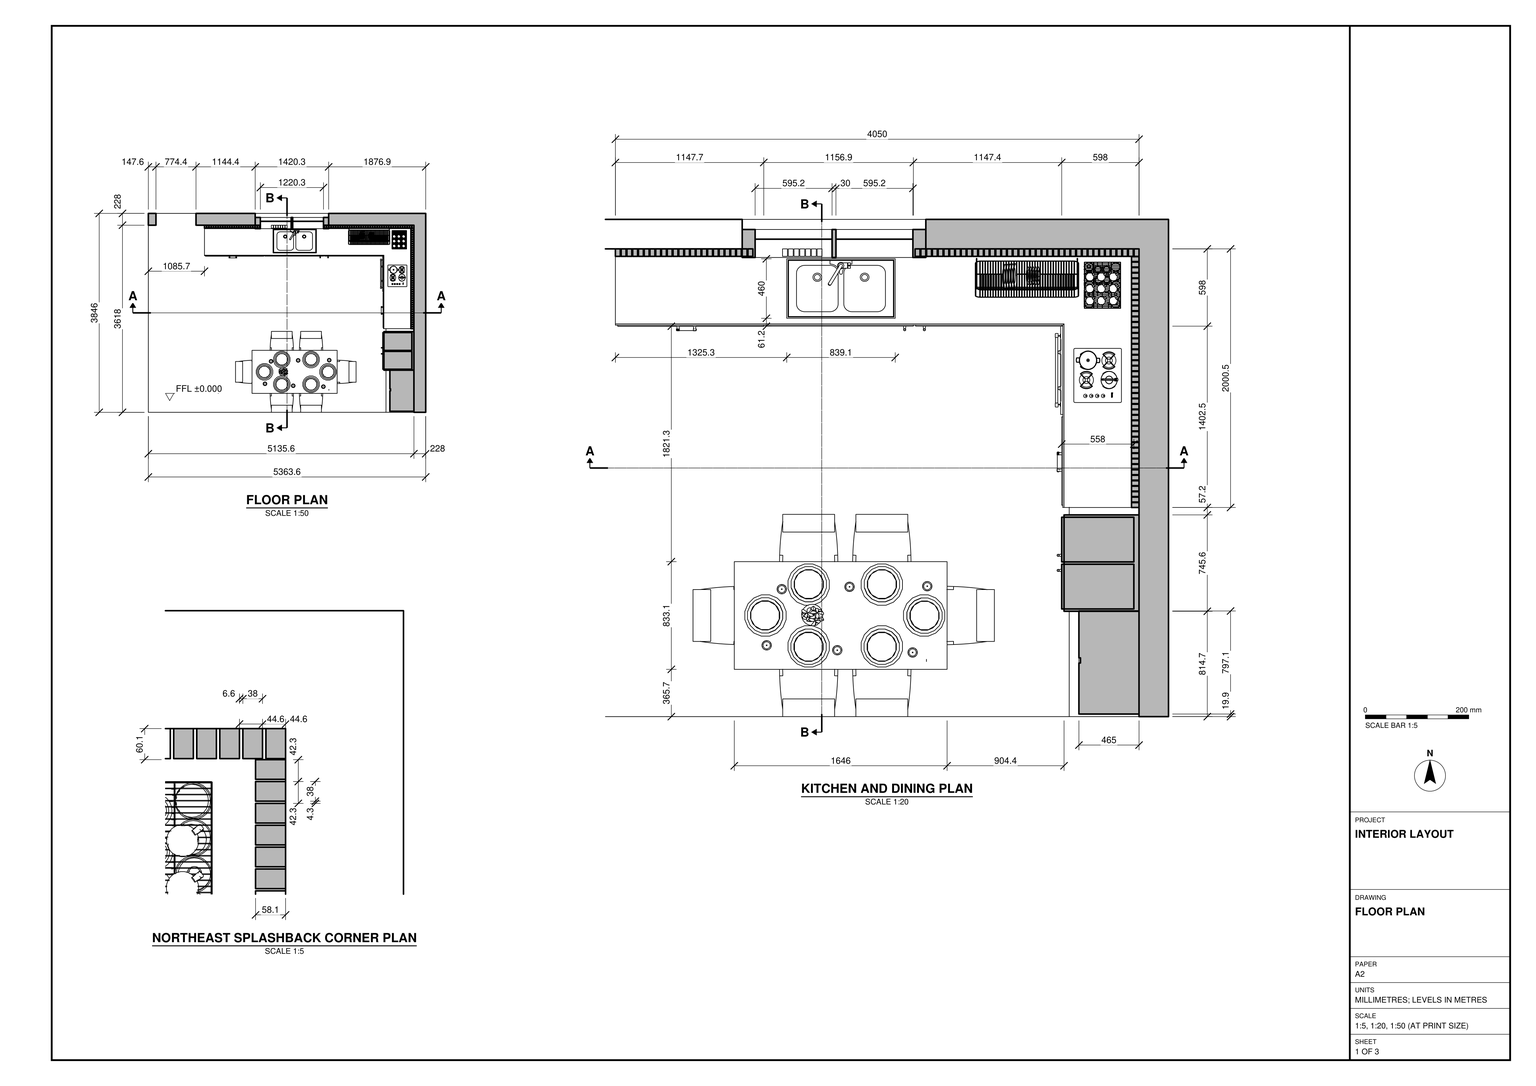
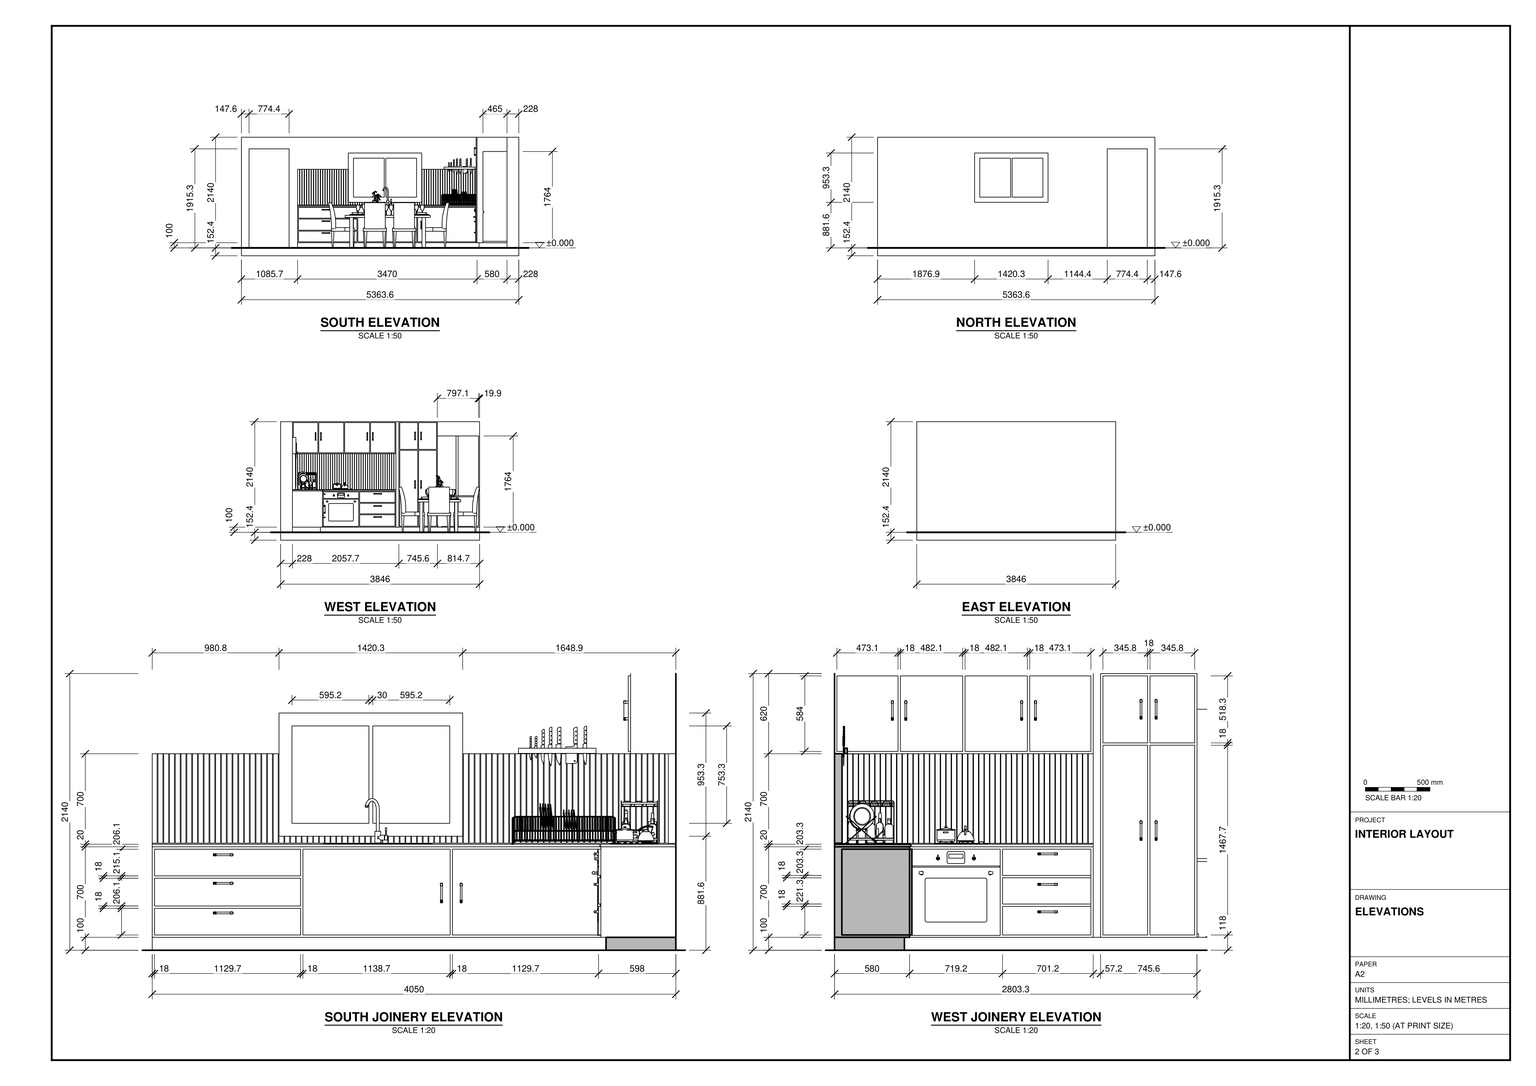
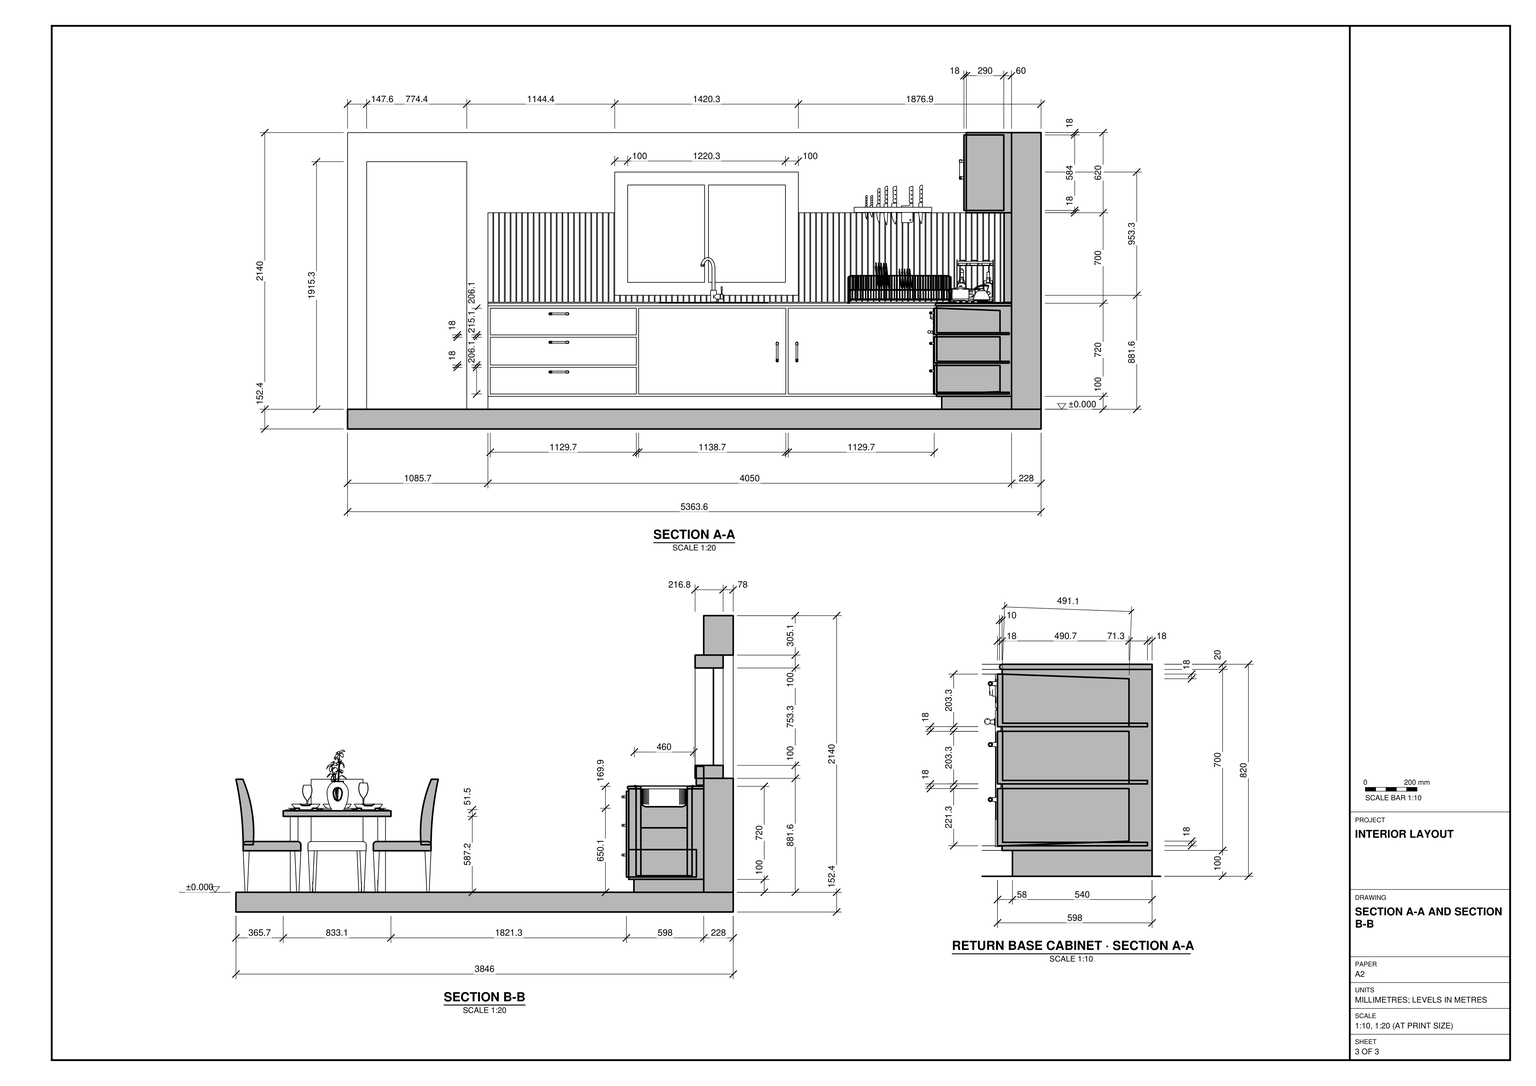
Build the kitchen and dining interior in SketchUp from task_files/diagram_01.pdf. Work in millimetres. The overall model measures 5363.6 mm east–west, 3846 mm north–south and 2292.4 mm high. Set the finished floor at 0 mm (±0.000), with the 152.4 mm slab below it. Build the 228 mm thick north and east walls to 2140 mm above the floor. Leave the south and west sides open as drawn.

Place the doorway near the west end of the north wall and the two-pane window above the double-bowl sink. Run the kitchen worktop along the north wall and turn it onto the east wall. Use the elevations and sections to lay out the plinths, drawer banks, cupboard fronts and handles. Model the vertically divided splashback around the corner, the wall cupboards above the east counter, the cooktop with the oven beneath it, and the tall storage and shallower end unit beyond the counter.

Place the rectangular dining table in the open area south of the sink, with chairs and place settings arranged as in plan. Decor, loose items and appliances may be any suitable library components. Keep the slab, walls and individual furniture and joinery pieces in separate groups or components, and use components for repeated parts. Save one SketchUp model as output_files/l_shaped_kitchen_and_six_seat_dining_area.skp.

# SketchUp Ruby script. Lengths in millimetres.
U = 1.mm
M = Sketchup.active_model
def pt(a) = Geom::Point3d.new(a.map { |v| v * U })
def face(e, loops, mat)
  f = e.add_face(loops[0].map { |a| pt(a) })
  loops[1..].each { |l| e.add_face(l.map { |a| pt(a) }).erase! }
  f.material = f.back_material = mat if mat
  f
end
# faces: each face lists its corners as indices into pts; further lists are holes
def faces(e, pts, list, mat = nil) = list.each { |f| face(e, (f[0].is_a?(Array) ? f : [f]).map { |l| l.map { |i| pts[i] } }, mat) }
# xy, xz, yz: faces in a plane at the given z, y or x. An outline is a flat list of corners, or four numbers for a rectangle; further outlines are holes
def ring(l) = l.size == 4 ? [[l[0], l[1]], [l[2], l[1]], [l[2], l[3]], [l[0], l[3]]] : l.each_slice(2).to_a
def flat(e, list, mat, &to3) = list.each { |f| face(e, (f[0].is_a?(Array) ? f : [f]).map { |l| ring(l).map { |u, v| to3.(u, v) } }, mat) }
def xy(e, z, list, mat = nil) = flat(e, list, mat) { |x, y| [x, y, z] }
def xz(e, y, list, mat = nil) = flat(e, list, mat) { |x, z| [x, y, z] }
def yz(e, x, list, mat = nil) = flat(e, list, mat) { |y, z| [x, y, z] }
def lines(e, pts, list) = list.each { |a, b| e.add_line(pt(pts[a]), pt(pts[b])) }
# prism: a flat outline (further loops are holes) pulled along v
def prism(e, loops, v, mat = nil)
  f = face(e, loops, mat); d = Geom::Vector3d.new(v.map { |x| x * U })
  f.pushpull(f.normal.samedirection?(d) ? d.length : -d.length)
end
def box(e, o, s, mat = nil) = prism(e, [[o, [o[0] + s[0], o[1], o[2]], [o[0] + s[0], o[1] + s[1], o[2]], [o[0], o[1] + s[1], o[2]]]], [0, 0, s[2]], mat)
def at(x, y, z, deg = 0) = Geom::Transformation.translation(pt([x, y, z])) * Geom::Transformation.rotation(ORIGIN, Z_AXIS, deg.degrees)
def axes(o, x, y, z) = Geom::Transformation.new([*x, 0, *y, 0, *z, 0, *pt(o).to_a, 1])
def part(name) = M.definitions.add(name)
# library, detail: a bought-in or finely detailed component or shape, given as its bounding box
def library(name, o, s) = part(name).tap { |d| box(d.entities, o, s) }
def detail(e, o, s) = box(e.add_group.entities, o, s)
def put(e, d, t, mat = nil) = e.add_instance(d, t).tap { |i| i.material = mat if mat }
def group(e, t, mat = nil) = e.add_group.tap { |g| g.transformation = t; g.material = mat if mat }.entities
root = M.entities
M.materials.add("[Tile Limestone Multi]").color = [199, 173, 118]
M.materials.add("[Tile Linen]").color = [182, 181, 151]
M.materials.add("[Translucent Glass Blue]").color = [100, 149, 237]
M.materials["[Translucent Glass Blue]"].alpha = 0.5
M.materials.add("[Wood Cherry Original]").color = [152, 86, 42]
M.materials.add("[Wood Veneer 02]").color = [190, 128, 91]
c1 = library("1-POIGNEE CLC2",[-77,-9.5,0],[154,19,36])
c2 = library("Component",[8875.7,1239.1,100],[2724.7,3533.3,1764])
c3 = library("CCO-2400",[7.6,-531.8,-1.1],[389.7,493,455.1])
c4 = library("1-FOUR H60 CLC2",[0,-37.4,0],[597,555.4,597])
c5 = library("1-TABLE DE CUISSON CLC2",[-290,-255,0],[580,510,32])
c6 = library("1-VASEFLEURS CLC2",[-125.3,-110.7,0],[251.1,203.7,506.3])
c7 = library("Dining Table",[1385.7,1461.4,0],[1819,2710.3,1016.7])
c8 = library("Group\#4",[0,0,-752.2],[4050,2000.5,772.2])
c9 = part("Group\#13")
xy(c9.entities,0,[[-580,0,0,683.2]])
xy(c9.entities,13.3,[[-560,20,0,663.2]])
xy(c9.entities,203.3,[[-580,0,0,0,0,20,-560,20,-560,663.2,0,663.2,0,683.2,-580,683.2]])
xz(c9.entities,0,[[-580,0,0,203.3]])
xz(c9.entities,20,[[-560,13.3,0,203.3]])
xz(c9.entities,663.2,[[-560,13.3,0,203.3]])
xz(c9.entities,683.2,[[-580,0,0,203.3]])
yz(c9.entities,-580,[[0,0,683.2,203.3]])
yz(c9.entities,-560,[[20,13.3,663.2,203.3]])
yz(c9.entities,0,[[0,0,683.2,0,683.2,203.3,663.2,203.3,663.2,13.3,20,13.3,20,203.3,0,203.3]])
c10 = part("Group48\#1")
xy(c10.entities,0,[[-610.2,-376.6,-15,376.6],[15,-376.6,610.2,376.6]],"[Translucent Glass Blue]")
c11 = part("Group47\#1")
xy(c11.entities,0,[[[-710.2,-476.6,710.2,476.6],[15,-376.6,610.2,376.6],[-610.2,-376.6,-15,376.6]]],"[Wood Cherry Original]")
xy(c11.entities,216.8,[[[-710.2,-476.6,710.2,476.6],[15,-376.6,610.2,376.6],[-610.2,-376.6,-15,376.6]]],"[Wood Cherry Original]")
xz(c11.entities,-476.6,[[-710.2,0,710.2,216.8]])
xz(c11.entities,-376.6,[[-610.2,0,-15,216.8],[15,0,610.2,216.8]],"[Wood Cherry Original]")
xz(c11.entities,376.6,[[-610.2,0,-15,216.8],[15,0,610.2,216.8]])
xz(c11.entities,476.6,[[-710.2,0,710.2,216.8]],"[Wood Cherry Original]")
yz(c11.entities,-710.2,[[-476.6,0,476.6,216.8]],"[Wood Cherry Original]")
yz(c11.entities,-610.2,[[-376.6,0,376.6,216.8]],"[Wood Cherry Original]")
yz(c11.entities,-15,[[-376.6,0,376.6,216.8]],"[Wood Cherry Original]")
yz(c11.entities,15,[[-376.6,0,376.6,216.8]],"[Wood Cherry Original]")
yz(c11.entities,610.2,[[-376.6,0,376.6,216.8]],"[Wood Cherry Original]")
yz(c11.entities,710.2,[[-476.6,0,476.6,216.8]],"[Wood Cherry Original]")
put(c11.entities,c10,at(0,0,75))
c12 = part("Group\#19")
box(c12.entities,[-18,0,0],[18,345.8,518.3])
c13 = part("Group\#76")
box(c13.entities,[-18,0,0],[18,345.8,1467.7])
p = [[2066.4,3618,881.6],[2066.4,3618,1834.9],[3486.8,3618,1834.9],[3486.8,3618,881.6]]
lines(root,p,[[0,1],[1,2],[2,3],[3,0]])
put(root,c1,axes([1634.5,3020,288.4],[1,0,0],[0,0,1],[0,-1,0]))
put(root,c1,axes([1634.5,3020,518],[1,0,0],[0,0,1],[0,-1,0]))
put(root,c1,axes([1634.5,3020,738.2],[1,0,0],[0,0,1],[0,-1,0]))
put(root,c1,axes([3323,3020,442.8],[0,0,1],[-1,0,0],[0,-1,0]))
put(root,c1,axes([3475.3,3020,442.8],[0,0,1],[-1,0,0],[0,-1,0]))
put(root,c1,axes([4537.7,1970.1,745.1],[0,-1,0],[0,0,1],[-1,0,0]))
put(root,c1,axes([4537.7,1970.1,509.4],[0,-1,0],[0,0,1],[-1,0,0]))
put(root,c1,axes([4537.7,1970.1,296.8],[0,-1,0],[0,0,1],[-1,0,0]))
put(root,c1,axes([4767.7,3170.8,1854.3],[0,0,1],[0,1,0],[-1,0,0]))
put(root,c1,axes([4767.7,3067,1854.3],[0,0,1],[0,1,0],[-1,0,0]))
put(root,c1,axes([4767.7,2171,1854.3],[0,0,1],[0,1,0],[-1,0,0]))
put(root,c1,axes([4767.7,2064,1854.3],[0,0,1],[0,1,0],[-1,0,0]))
put(root,c2,at(-6464.7,-1219.1,0))
put(root,c3,axes([4700,3550.8,820.8],[0.74,0,0],[0,0.74,0],[0,0,0.74]))
put(root,c1,axes([4537.6,1247.7,1863.7],[0,0,1],[0,1,0],[-1,0,0]))
put(root,c1,axes([4537.6,1130.9,1863.7],[0,0,1],[0,1,0],[-1,0,0]))
put(root,c1,axes([4537.6,1130.9,925.8],[0,0,1],[0,1,0],[-1,0,0]))
put(root,c1,axes([4537.6,1247.7,925.8],[0,0,1],[0,1,0],[-1,0,0]))
put(root,c4,axes([4529.6,3020,114.7],[0,-1.14447,0],[1.1224,0,0],[0,0,1.11769]))
put(root,c5,axes([4815.5,2638.8,820],[0,-0.7221,0],[0.7221,0,0],[0,0,0.7221]))
put(root,c6,at(2607.9,785.6,629.8))
put(root,c7,axes([5273.7,-1191.7,0],[0,0.86,0],[-0.86,0,0],[0,0,0.86]))
g1 = group(root,at(1085.6,0,0))
prism(g1,[[[3510,3078,0],[0,3078,0],[0,3618,0],[4050,3618,0],[4050,0,0],[3510,0,0]]],[0,0,100])
g2 = group(root,at(4555.6,10.3,100),"[Wood Veneer 02]")
xy(g2,0,[[0,804.4,580,1550]])
xy(g2,18,[[0,822.4,540,1168.2],[0,1186.2,540,1532]])
xy(g2,1485.7,[[0,822.4,540,1168.2],[0,1186.2,540,1532]])
xy(g2,1503.7,[[0,822.4,540,1168.2],[0,1186.2,540,1532]])
xy(g2,2022,[[0,822.4,540,1168.2],[0,1186.2,540,1532]])
xy(g2,2040,[[0,804.4,580,1550]])
xz(g2,804.4,[[0,0,580,2040]])
xz(g2,822.4,[[0,18,540,1485.7],[0,1503.7,540,2022]])
xz(g2,1168.2,[[0,18,540,1485.7],[0,1503.7,540,2022]])
xz(g2,1186.2,[[0,18,540,1485.7],[0,1503.7,540,2022]])
xz(g2,1532,[[0,18,540,1485.7],[0,1503.7,540,2022]])
xz(g2,1550,[[0,0,580,2040]])
yz(g2,0,[[[804.4,0,1550,2040],[822.4,18,1168.2,1485.7],[1186.2,18,1532,1485.7],[822.4,1503.7,1168.2,2022],[1186.2,1503.7,1532,2022]]])
yz(g2,540,[[822.4,18,1168.2,1485.7],[1186.2,18,1532,1485.7],[822.4,1503.7,1168.2,2022],[1186.2,1503.7,1532,2022]])
yz(g2,580,[[804.4,0,1550,2040]])
g3 = group(root,at(1085.6,1617.5,100))
xy(g3,0,[[3470,0,3470,1420.5,0,1420.5,0,2000.5,4050,2000.5,4050,0]])
xy(g3,18,[[3470,719.2,3960.7,1402.5],[18,1420.5,1147.7,1944],[1165.7,1420.5,2304.3,1944],[2322.3,1420.5,3452,1944]])
xy(g3,224.1,[[18,1420.5,1147.7,1944]])
xy(g3,230.1,[[1165.7,1420.5,2304.3,1944]])
xy(g3,239.3,[[3470,18,3960.7,701.2]])
xy(g3,242.1,[[18,1420.5,1147.7,1944]])
xy(g3,257.3,[[3470,18,3960.7,701.2]])
xy(g3,457.2,[[18,1420.5,1147.7,1944]])
xy(g3,460.7,[[3470,18,3960.7,701.2]])
xy(g3,475.2,[[18,1420.5,1147.7,1944]])
xy(g3,478.7,[[3470,18,3960.7,701.2]])
xy(g3,682,[[3470,719.2,3960.7,1402.5],[18,1420.5,1147.7,1944],[2322.3,1420.5,3452,1944]])
xz(g3,0,[[3470,0,4050,700]],"[Wood Veneer 02]")
xz(g3,18,[[3470,18,3470,239.3,3960.7,239.3,3960.7,36],[3470,257.3,3960.7,460.7],[3470,478.7,3470,682,3960.7,664,3960.7,478.7]])
xz(g3,701.2,[[3470,18,3960.7,36,3960.7,239.3,3470,239.3],[3470,257.3,3960.7,460.7],[3470,478.7,3960.7,478.7,3960.7,664,3470,682]])
xz(g3,719.2,[[3470,18,3960.7,682]])
xz(g3,1402.5,[[3470,18,3960.7,682]])
xz(g3,1420.5,[[[0,0,3470,700],[2322.3,18,3452,682],[18,242.1,1147.7,457.2],[1165.7,18,2304.3,230.1],[18,475.2,1147.7,682],[18,18,1147.7,224.1]]],"[Wood Veneer 02]")
xz(g3,1944,[[18,18,1147.7,224.1],[1165.7,18,2304.3,230.1],[2322.3,18,3452,682],[18,242.1,1147.7,457.2],[18,475.2,1147.7,682]])
xz(g3,2000.5,[[0,0,4050,700]])
yz(g3,0,[[1420.5,0,2000.5,700]],"[Wood Veneer 02]")
yz(g3,18,[[1420.5,18,1944,224.1],[1420.5,242.1,1944,457.2],[1420.5,475.2,1944,682]])
yz(g3,1147.7,[[1420.5,18,1944,224.1],[1420.5,242.1,1944,457.2],[1420.5,475.2,1944,682]])
yz(g3,1165.7,[[1420.5,18,1944,230.1]])
yz(g3,2304.3,[[1420.5,18,1944,230.1]])
yz(g3,2322.3,[[1420.5,18,1944,682]])
yz(g3,3452,[[1420.5,18,1944,682]])
yz(g3,3470,[[[0,0,1420.5,700],[719.2,18,1402.5,682],[18,18,701.2,18,701.2,239.3,18,239.3,18,257.3,701.2,257.3,701.2,460.7,18,460.7,18,478.7,701.2,478.7,701.2,682,18,682]]],"[Wood Veneer 02]")
yz(g3,3960.7,[[719.2,18,1402.5,682],[18,36,701.2,239.3],[18,257.3,701.2,460.7],[18,478.7,701.2,664]])
yz(g3,4050,[[0,0,2000.5,700]])
p = [[3470,701.2,18],[3470,18,18],[3960.7,18,36],[3960.7,701.2,36],[3470,18,682],[3470,701.2,682],
  [3960.7,701.2,664],[3960.7,18,664]]
faces(g3,p,[[0,1,2,3],[4,5,6,7]])
put(g3,c8,at(0,0,700))
g4 = group(g3,at(18.3,1982.5,18),"[Wood Veneer 02]")
xy(g4,0,[[0,-580,1129.7,0]])
xy(g4,0.5,[[60.9,-519.1,1068.8,0]])
xy(g4,206.1,[[0,-580,1129.7,-580,1129.7,0,1068.8,0,1068.8,-519.1,60.9,-519.1,60.9,0,0,0]])
xz(g4,-580,[[0,0,1129.7,206.1]])
xz(g4,-519.1,[[60.9,0.5,1068.8,206.1]])
xz(g4,0,[[0,0,0,206.1,60.9,206.1,60.9,0.5,1068.8,0.5,1068.8,206.1,1129.7,206.1,1129.7,0]])
yz(g4,0,[[-580,0,0,206.1]])
yz(g4,60.9,[[-519.1,0.5,0,206.1]])
yz(g4,1068.8,[[-519.1,0.5,0,206.1]])
yz(g4,1129.7,[[-580,0,0,206.1]])
g5 = group(g3,at(18,1982.5,242.1),"[Wood Veneer 02]")
xy(g5,0,[[0,-580,1129.7,0]])
xy(g5,0.5,[[60.9,-519.1,1068.8,0]])
xy(g5,215.1,[[0,-580,1129.7,-580,1129.7,0,1068.8,0,1068.8,-519.1,60.9,-519.1,60.9,0,0,0]])
xz(g5,-580,[[0,0,1129.7,215.1]])
xz(g5,-519.1,[[60.9,0.5,1068.8,215.1]])
xz(g5,0,[[0,0,0,215.1,60.9,215.1,60.9,0.5,1068.8,0.5,1068.8,215.1,1129.7,215.1,1129.7,0]])
yz(g5,0,[[-580,0,0,215.1]])
yz(g5,60.9,[[-519.1,0.5,0,215.1]])
yz(g5,1068.8,[[-519.1,0.5,0,215.1]])
yz(g5,1129.7,[[-580,0,0,215.1]])
g6 = group(g3,at(18,1981.1,475.2),"[Wood Veneer 02]")
xy(g6,0,[[0,-580,1129.7,0]])
xy(g6,0.5,[[60.9,-519.1,1068.8,0]])
xy(g6,206.1,[[0,-580,1129.7,-580,1129.7,0,1068.8,0,1068.8,-519.1,60.9,-519.1,60.9,0,0,0]])
xz(g6,-580,[[0,0,1129.7,206.1]])
xz(g6,-519.1,[[60.9,0.5,1068.8,206.1]])
xz(g6,0,[[0,0,0,206.1,60.9,206.1,60.9,0.5,1068.8,0.5,1068.8,206.1,1129.7,206.1,1129.7,0]])
yz(g6,0,[[-580,0,0,206.1]])
yz(g6,60.9,[[-519.1,0.5,0,206.1]])
yz(g6,1068.8,[[-519.1,0.5,0,206.1]])
yz(g6,1129.7,[[-580,0,0,206.1]])
g7 = group(root,at(4785.6,1617.5,1520))
xy(g7,0,[[0,0,350,2000.5]])
xy(g7,18,[[0,18,290,491.1],[0,509.1,290,991.2],[0,1009.2,290,1491.4],[0,1509.4,290,1982.5]])
xy(g7,602,[[0,18,290,491.1],[0,509.1,290,991.2],[0,1009.2,290,1491.4],[0,1509.4,290,1982.5]])
xy(g7,620,[[0,0,350,2000.5]])
xz(g7,0,[[0,0,350,620]])
xz(g7,18,[[0,18,290,602]])
xz(g7,491.1,[[0,18,290,602]])
xz(g7,509.1,[[0,18,290,602]])
xz(g7,991.2,[[0,18,290,602]])
xz(g7,1009.2,[[0,18,290,602]])
xz(g7,1491.4,[[0,18,290,602]])
xz(g7,1509.4,[[0,18,290,602]])
xz(g7,1982.5,[[0,18,290,602]])
xz(g7,2000.5,[[0,0,350,620]])
yz(g7,0,[[[0,0,2000.5,620],[509.1,18,991.2,602],[1009.2,18,1491.4,602],[18,18,491.1,602],[1509.4,18,1982.5,602]]])
yz(g7,290,[[18,18,491.1,602],[509.1,18,991.2,602],[1009.2,18,1491.4,602],[1509.4,18,1982.5,602]])
yz(g7,350,[[0,0,2000.5,620]])
g8 = group(root,at(1085.6,1617.5,820),"[Tile Linen]")
box(g8,[0,1942.4,8.1],[38,58.1,691.9])
box(g8,[44.6,1942.4,8.1],[38,58.1,691.9])
box(g8,[89.2,1942.4,8.1],[38,58.1,691.9])
box(g8,[133.7,1942.4,8.1],[38.1,58.1,691.9])
box(g8,[178.3,1942.4,8.1],[38,58.1,691.9])
box(g8,[222.9,1942.4,8.1],[38,58.1,691.9])
box(g8,[267.5,1942.4,8.1],[38,58.1,691.9])
box(g8,[312,1942.4,8.1],[38.1,58.1,691.9])
box(g8,[356.6,1942.4,8.1],[38,58.1,691.9])
box(g8,[401.2,1942.4,8.1],[38,58.1,691.9])
box(g8,[445.8,1942.4,8.1],[38,58.1,691.9])
box(g8,[490.4,1942.4,8.1],[38,58.1,691.9])
box(g8,[534.9,1942.4,8.1],[38.1,58.1,691.9])
box(g8,[579.5,1942.4,8.1],[38,58.1,691.9])
box(g8,[624.1,1942.4,8.1],[38,58.1,691.9])
box(g8,[668.7,1942.4,8.1],[38,58.1,691.9])
box(g8,[713.2,1942.4,8.1],[38.1,58.1,691.9])
box(g8,[757.8,1942.4,8.1],[38,58.1,691.9])
box(g8,[802.4,1942.4,8.1],[38,58.1,691.9])
box(g8,[847,1942.4,8.1],[38,58.1,691.9])
box(g8,[891.6,1942.4,8.1],[38,58.1,691.9])
box(g8,[936.1,1942.4,8.1],[38,58.1,691.9])
box(g8,[980.7,1942.4,8.1],[38,58.1,691.9])
box(g8,[1025.3,1942.4,8.1],[38,58.1,691.9])
box(g8,[1069.9,1942.4,8.1],[38,58.1,89.3])
box(g8,[1114.4,1942.4,8.1],[38.1,58.1,53.5])
box(g8,[1159,1942.4,8.1],[38,58.1,97.8])
box(g8,[1248.2,1942.4,8.1],[38,58.1,53.5])
box(g8,[1292.7,1942.4,8.1],[38.1,58.1,146.3])
box(g8,[1337.3,1942.4,8.1],[38,58.1,146.3])
box(g8,[1381.9,1942.4,8.1],[38,58.1,146.3])
box(g8,[1426.5,1942.4,8.1],[38,58.1,146.3])
box(g8,[1471.1,1942.4,8.1],[38,58.1,146.3])
box(g8,[1515.6,1942.4,8.1],[38.1,58.1,146.3])
box(g8,[1560.2,1942.4,8.1],[38,58.1,146.3])
box(g8,[1604.8,1942.4,8.1],[38,58.1,53.5])
box(g8,[1649.4,1942.4,8.1],[38,58.1,54.1])
box(g8,[1693.9,1942.4,8.1],[38.1,58.1,53.5])
box(g8,[1738.5,1942.4,8.1],[38,58.1,53.5])
box(g8,[1783.1,1942.4,8.1],[38,58.1,76.2])
box(g8,[1827.7,1942.4,8.1],[38,58.1,76.2])
box(g8,[1872.3,1942.4,8.1],[38,58.1,76.2])
box(g8,[1916.8,1942.4,8.1],[38.1,58.1,76.2])
box(g8,[1961.4,1942.4,8.1],[38,58.1,76.2])
box(g8,[2006,1942.4,8.1],[38,58.1,76.2])
box(g8,[2050.6,1942.4,8.1],[38,58.1,76.2])
box(g8,[2095.1,1942.4,8.1],[38.1,58.1,76.2])
box(g8,[2139.7,1942.4,8.1],[38,58.1,76.2])
box(g8,[2184.3,1942.4,8.1],[38,58.1,76.2])
box(g8,[2228.9,1942.4,8.1],[38,58.1,76.2])
box(g8,[2273.5,1942.4,8.1],[38,58.1,76.2])
box(g8,[2318,1942.4,8.1],[38.1,58.1,691.9])
box(g8,[2362.6,1942.4,8.1],[38,58.1,691.9])
box(g8,[2407.2,1942.4,8.1],[38,58.1,691.9])
box(g8,[2451.8,1942.4,8.1],[38,58.1,691.9])
box(g8,[2496.3,1942.4,8.1],[38.1,58.1,691.9])
box(g8,[2540.9,1942.4,8.1],[38,58.1,691.9])
box(g8,[2585.5,1942.4,8.1],[38,58.1,691.9])
box(g8,[2630.1,1942.4,8.1],[38,58.1,691.9])
box(g8,[2674.7,1942.4,8.1],[38,58.1,691.9])
box(g8,[2719.2,1942.4,8.1],[38.1,58.1,691.9])
box(g8,[2763.8,1942.4,8.1],[38,58.1,691.9])
box(g8,[2808.4,1942.4,8.1],[38,58.1,691.9])
box(g8,[2853,1942.4,8.1],[38,58.1,691.9])
box(g8,[2897.5,1942.4,8.1],[38.1,58.1,691.9])
box(g8,[2942.1,1942.4,8.1],[38,58.1,691.9])
box(g8,[2986.7,1942.4,8.1],[38,58.1,691.9])
box(g8,[3031.3,1942.4,8.1],[38,58.1,691.9])
box(g8,[3075.9,1942.4,8.1],[38,58.1,691.9])
box(g8,[3120.4,1942.4,8.1],[38,58.1,691.9])
box(g8,[3165,1942.4,8.1],[38,58.1,691.9])
box(g8,[3209.6,1942.4,8.1],[38,58.1,691.9])
box(g8,[3254.2,1942.4,8.1],[38,58.1,691.9])
box(g8,[3298.7,1942.4,8.1],[38.1,58.1,691.9])
box(g8,[3343.3,1942.4,8.1],[38,58.1,691.9])
box(g8,[3387.9,1942.4,8.1],[38,58.1,691.9])
box(g8,[3432.5,1942.4,8.1],[38,58.1,691.9])
box(g8,[3477,1942.4,8.1],[38.1,58.1,691.9])
box(g8,[3521.6,1942.4,8.1],[38,58.1,691.9])
box(g8,[3566.2,1942.4,8.1],[38,58.1,691.9])
box(g8,[3610.8,1942.4,8.1],[38,58.1,691.9])
box(g8,[3655.4,1942.4,8.1],[38,58.1,691.9])
box(g8,[3699.9,1942.4,8.1],[38.1,58.1,691.9])
box(g8,[3744.5,1942.4,8.1],[38,58.1,691.9])
box(g8,[3789.1,1942.4,8.1],[38,58.1,691.9])
box(g8,[3833.7,1942.4,8.1],[38,58.1,691.9])
box(g8,[3878.2,1942.4,8.1],[38.1,58.1,691.9])
box(g8,[3922.8,1942.4,8.1],[38,58.1,691.9])
box(g8,[3967.4,1942.4,8.1],[38,58.1,691.9])
box(g8,[3991.9,1733.3,6.8],[58.1,38,691.9])
box(g8,[3991.9,1775.6,6.8],[58.1,38,691.9])
box(g8,[3991.9,1817.8,6.8],[58.1,38.1,691.9])
box(g8,[3991.9,1860.1,6.8],[58.1,38,691.9])
box(g8,[3991.9,1902.4,6.8],[58.1,38,691.9])
box(g8,[1203.6,1942.4,8.1],[38,58.1,53.5])
xy(g8,6.8,[[3991.9,0,4050,38],[3991.9,42.3,4050,80.3],[3991.9,84.6,4050,122.6],[3991.9,126.8,4050,164.8],[3991.9,169.1,4050,207.1],
  [3991.9,211.4,4050,249.4],[3991.9,253.7,4050,291.7],[3991.9,295.9,4050,333.9],[3991.9,338.2,4050,376.2],[3991.9,380.5,4050,418.5],
  [3991.9,422.8,4050,460.8],[3991.9,465,4050,503.1],[3991.9,507.3,4050,545.3],[3991.9,549.6,4050,587.6],[3991.9,591.9,4050,629.9],
  [3991.9,634.1,4050,672.2],[3991.9,676.4,4050,714.4],[3991.9,718.7,4050,756.7],[3991.9,761,4050,799],[3991.9,803.2,4050,841.3],
  [3991.9,845.5,4050,883.5],[3991.9,887.8,4050,925.8],[3991.9,930.1,4050,968.1],[3991.9,972.3,4050,1010.4],[3991.9,1014.6,4050,1052.6],
  [3991.9,1056.9,4050,1094.9],[3991.9,1099.2,4050,1137.2],[3991.9,1141.4,4050,1179.5],[3991.9,1183.7,4050,1221.7],[3991.9,1226,4050,1264],
  [3991.9,1268.3,4050,1306.3],[3991.9,1310.5,4050,1348.6],[3991.9,1352.8,4050,1390.8],[3991.9,1395.1,4050,1433.1],[3991.9,1437.4,4050,1475.4],
  [3991.9,1479.6,4050,1517.7],[3991.9,1521.9,4050,1559.9],[3991.9,1564.2,4050,1602.2],[3991.9,1606.5,4050,1644.5],[3991.9,1648.7,4050,1686.8],
  [3991.9,1691,4050,1729]])
xy(g8,8.1,[[4012,1942.4,4050,2000.5]])
xy(g8,700,[[3991.9,0,4050,38],[3991.9,42.3,4050,80.3],[3991.9,84.6,4050,122.6],[3991.9,126.8,4050,164.8],[3991.9,169.1,4050,207.1],
  [3991.9,211.4,4050,249.4],[3991.9,253.7,4050,291.7],[3991.9,295.9,4050,333.9],[3991.9,338.2,4050,376.2],[3991.9,380.5,4050,418.5],
  [3991.9,422.8,4050,460.8],[3991.9,465,4050,503.1],[3991.9,507.3,4050,545.3],[3991.9,549.6,4050,587.6],[3991.9,591.9,4050,629.9],
  [3991.9,634.1,4050,672.2],[3991.9,676.4,4050,714.4],[3991.9,718.7,4050,756.7],[3991.9,761,4050,799],[3991.9,803.2,4050,841.3],
  [3991.9,845.5,4050,883.5],[3991.9,887.8,4050,925.8],[3991.9,930.1,4050,968.1],[3991.9,972.3,4050,1010.4],[3991.9,1014.6,4050,1052.6],
  [3991.9,1056.9,4050,1094.9],[3991.9,1099.2,4050,1137.2],[3991.9,1141.4,4050,1179.5],[3991.9,1183.7,4050,1221.7],[3991.9,1226,4050,1264],
  [3991.9,1268.3,4050,1306.3],[3991.9,1310.5,4050,1348.6],[3991.9,1352.8,4050,1390.8],[3991.9,1395.1,4050,1433.1],[3991.9,1437.4,4050,1475.4],
  [3991.9,1479.6,4050,1517.7],[3991.9,1521.9,4050,1559.9],[3991.9,1564.2,4050,1602.2],[3991.9,1606.5,4050,1644.5],[3991.9,1648.7,4050,1686.8],
  [3991.9,1691,4050,1729],[4012,1942.4,4050,2000.5]])
xz(g8,0,[[3991.9,6.8,4050,700]])
xz(g8,38,[[3991.9,6.8,4050,700]])
xz(g8,42.3,[[3991.9,6.8,4050,700]])
xz(g8,80.3,[[3991.9,6.8,4050,700]])
xz(g8,84.6,[[3991.9,6.8,4050,700]])
xz(g8,122.6,[[3991.9,6.8,4050,700]])
xz(g8,126.8,[[3991.9,6.8,4050,700]])
xz(g8,164.8,[[3991.9,6.8,4050,700]])
xz(g8,169.1,[[3991.9,6.8,4050,700]])
xz(g8,207.1,[[3991.9,6.8,4050,700]])
xz(g8,211.4,[[3991.9,6.8,4050,700]])
xz(g8,249.4,[[3991.9,6.8,4050,700]])
xz(g8,253.7,[[3991.9,6.8,4050,700]])
xz(g8,291.7,[[3991.9,6.8,4050,700]])
xz(g8,295.9,[[3991.9,6.8,4050,700]])
xz(g8,333.9,[[3991.9,6.8,4050,700]])
xz(g8,338.2,[[3991.9,6.8,4050,700]])
xz(g8,376.2,[[3991.9,6.8,4050,700]])
xz(g8,380.5,[[3991.9,6.8,4050,700]])
xz(g8,418.5,[[3991.9,6.8,4050,700]])
xz(g8,422.8,[[3991.9,6.8,4050,700]])
xz(g8,460.8,[[3991.9,6.8,4050,700]])
xz(g8,465,[[3991.9,6.8,4050,700]])
xz(g8,503.1,[[3991.9,6.8,4050,700]])
xz(g8,507.3,[[3991.9,6.8,4050,700]])
xz(g8,545.3,[[3991.9,6.8,4050,700]])
xz(g8,549.6,[[3991.9,6.8,4050,700]])
xz(g8,587.6,[[3991.9,6.8,4050,700]])
xz(g8,591.9,[[3991.9,6.8,4050,700]])
xz(g8,629.9,[[3991.9,6.8,4050,700]])
xz(g8,634.1,[[3991.9,6.8,4050,700]])
xz(g8,672.2,[[3991.9,6.8,4050,700]])
xz(g8,676.4,[[3991.9,6.8,4050,700]])
xz(g8,714.4,[[3991.9,6.8,4050,700]])
xz(g8,718.7,[[3991.9,6.8,4050,700]])
xz(g8,756.7,[[3991.9,6.8,4050,700]])
xz(g8,761,[[3991.9,6.8,4050,700]])
xz(g8,799,[[3991.9,6.8,4050,700]])
xz(g8,803.2,[[3991.9,6.8,4050,700]])
xz(g8,841.3,[[3991.9,6.8,4050,700]])
xz(g8,845.5,[[3991.9,6.8,4050,700]])
xz(g8,883.5,[[3991.9,6.8,4050,700]])
xz(g8,887.8,[[3991.9,6.8,4050,700]])
xz(g8,925.8,[[3991.9,6.8,4050,700]])
xz(g8,930.1,[[3991.9,6.8,4050,700]])
xz(g8,968.1,[[3991.9,6.8,4050,700]])
xz(g8,972.3,[[3991.9,6.8,4050,700]])
xz(g8,1010.4,[[3991.9,6.8,4050,700]])
xz(g8,1014.6,[[3991.9,6.8,4050,700]])
xz(g8,1052.6,[[3991.9,6.8,4050,700]])
xz(g8,1056.9,[[3991.9,6.8,4050,700]])
xz(g8,1094.9,[[3991.9,6.8,4050,700]])
xz(g8,1099.2,[[3991.9,6.8,4050,700]])
xz(g8,1137.2,[[3991.9,6.8,4050,700]])
xz(g8,1141.4,[[3991.9,6.8,4050,700]])
xz(g8,1179.5,[[3991.9,6.8,4050,700]])
xz(g8,1183.7,[[3991.9,6.8,4050,700]])
xz(g8,1221.7,[[3991.9,6.8,4050,700]])
xz(g8,1226,[[3991.9,6.8,4050,700]])
xz(g8,1264,[[3991.9,6.8,4050,700]])
xz(g8,1268.3,[[3991.9,6.8,4050,700]])
xz(g8,1306.3,[[3991.9,6.8,4050,700]])
xz(g8,1310.5,[[3991.9,6.8,4050,700]])
xz(g8,1348.6,[[3991.9,6.8,4050,700]])
xz(g8,1352.8,[[3991.9,6.8,4050,700]])
xz(g8,1390.8,[[3991.9,6.8,4050,700]])
xz(g8,1395.1,[[3991.9,6.8,4050,700]])
xz(g8,1433.1,[[3991.9,6.8,4050,700]])
xz(g8,1437.4,[[3991.9,6.8,4050,700]])
xz(g8,1475.4,[[3991.9,6.8,4050,700]])
xz(g8,1479.6,[[3991.9,6.8,4050,700]])
xz(g8,1517.7,[[3991.9,6.8,4050,700]])
xz(g8,1521.9,[[3991.9,6.8,4050,700]])
xz(g8,1559.9,[[3991.9,6.8,4050,700]])
xz(g8,1564.2,[[3991.9,6.8,4050,700]])
xz(g8,1602.2,[[3991.9,6.8,4050,700]])
xz(g8,1606.5,[[3991.9,6.8,4050,700]])
xz(g8,1644.5,[[3991.9,6.8,4050,700]])
xz(g8,1648.7,[[3991.9,6.8,4050,700]])
xz(g8,1686.8,[[3991.9,6.8,4050,700]])
xz(g8,1691,[[3991.9,6.8,4050,700]])
xz(g8,1729,[[3991.9,6.8,4050,700]])
xz(g8,1942.4,[[4012,8.1,4050,700]])
xz(g8,2000.5,[[4012,8.1,4050,700]])
yz(g8,3991.9,[[0,6.8,38,700],[42.3,6.8,80.3,700],[84.6,6.8,122.6,700],[126.8,6.8,164.8,700],[169.1,6.8,207.1,700],
  [211.4,6.8,249.4,700],[253.7,6.8,291.7,700],[295.9,6.8,333.9,700],[338.2,6.8,376.2,700],[380.5,6.8,418.5,700],
  [422.8,6.8,460.8,700],[465,6.8,503.1,700],[507.3,6.8,545.3,700],[549.6,6.8,587.6,700],[591.9,6.8,629.9,700],
  [634.1,6.8,672.2,700],[676.4,6.8,714.4,700],[718.7,6.8,756.7,700],[761,6.8,799,700],[803.2,6.8,841.3,700],
  [845.5,6.8,883.5,700],[887.8,6.8,925.8,700],[930.1,6.8,968.1,700],[972.3,6.8,1010.4,700],[1014.6,6.8,1052.6,700],
  [1056.9,6.8,1094.9,700],[1099.2,6.8,1137.2,700],[1141.4,6.8,1179.5,700],[1183.7,6.8,1221.7,700],[1226,6.8,1264,700],
  [1268.3,6.8,1306.3,700],[1310.5,6.8,1348.6,700],[1352.8,6.8,1390.8,700],[1395.1,6.8,1433.1,700],[1437.4,6.8,1475.4,700],
  [1479.6,6.8,1517.7,700],[1521.9,6.8,1559.9,700],[1564.2,6.8,1602.2,700],[1606.5,6.8,1644.5,700],[1648.7,6.8,1686.8,700],
  [1691,6.8,1729,700]])
yz(g8,4012,[[1942.4,8.1,2000.5,700]])
yz(g8,4050,[[0,0,2000.5,0,2000.5,8.1,1942.4,8.1,1942.4,700,1729,700,1729,6.8,1691,6.8,1691,700,1686.8,700,1686.8,6.8,1648.7,6.8,1648.7,700,1644.5,700,1644.5,6.8,1606.5,6.8,1606.5,700,1602.2,700,1602.2,6.8,1564.2,6.8,1564.2,700,1559.9,700,1559.9,6.8,1521.9,6.8,1521.9,700,1517.7,700,1517.7,6.8,1479.6,6.8,1479.6,700,1475.4,700,1475.4,6.8,1437.4,6.8,1437.4,700,1433.1,700,1433.1,6.8,1395.1,6.8,1395.1,700,1390.8,700,1390.8,6.8,1352.8,6.8,1352.8,700,1348.6,700,1348.6,6.8,1310.5,6.8,1310.5,700,1306.3,700,1306.3,6.8,1268.3,6.8,1268.3,700,1264,700,1264,6.8,1226,6.8,1226,700,1221.7,700,1221.7,6.8,1183.7,6.8,1183.7,700,1179.5,700,1179.5,6.8,1141.4,6.8,1141.4,700,1137.2,700,1137.2,6.8,1099.2,6.8,1099.2,700,1094.9,700,1094.9,6.8,1056.9,6.8,1056.9,700,1052.6,700,1052.6,6.8,1014.6,6.8,1014.6,700,1010.4,700,1010.4,6.8,972.3,6.8,972.3,700,968.1,700,968.1,6.8,930.1,6.8,930.1,700,925.8,700,925.8,6.8,887.8,6.8,887.8,700,883.5,700,883.5,6.8,845.5,6.8,845.5,700,841.3,700,841.3,6.8,803.2,6.8,803.2,700,799,700,799,6.8,761,6.8,761,700,756.7,700,756.7,6.8,718.7,6.8,718.7,700,714.4,700,714.4,6.8,676.4,6.8,676.4,700,672.2,700,672.2,6.8,634.1,6.8,634.1,700,629.9,700,629.9,6.8,591.9,6.8,591.9,700,587.6,700,587.6,6.8,549.6,6.8,549.6,700,545.3,700,545.3,6.8,507.3,6.8,507.3,700,503.1,700,503.1,6.8,465,6.8,465,700,460.8,700,460.8,6.8,422.8,6.8,422.8,700,418.5,700,418.5,6.8,380.5,6.8,380.5,700,376.2,700,376.2,6.8,338.2,6.8,338.2,700,333.9,700,333.9,6.8,295.9,6.8,295.9,700,291.7,700,291.7,6.8,253.7,6.8,253.7,700,249.4,700,249.4,6.8,211.4,6.8,211.4,700,207.1,700,207.1,6.8,169.1,6.8,169.1,700,164.8,700,164.8,6.8,126.8,6.8,126.8,700,122.6,700,122.6,6.8,84.6,6.8,84.6,700,80.3,700,80.3,6.8,42.3,6.8,42.3,700,38,700,38,6.8,0,6.8],[0,6.8,38,700],[42.3,6.8,80.3,700],[84.6,6.8,122.6,700],[126.8,6.8,164.8,700],
  [169.1,6.8,207.1,700],[211.4,6.8,249.4,700],[253.7,6.8,291.7,700],[295.9,6.8,333.9,700],[338.2,6.8,376.2,700],
  [380.5,6.8,418.5,700],[422.8,6.8,460.8,700],[465,6.8,503.1,700],[507.3,6.8,545.3,700],[549.6,6.8,587.6,700],
  [591.9,6.8,629.9,700],[634.1,6.8,672.2,700],[676.4,6.8,714.4,700],[718.7,6.8,756.7,700],[761,6.8,799,700],
  [803.2,6.8,841.3,700],[845.5,6.8,883.5,700],[887.8,6.8,925.8,700],[930.1,6.8,968.1,700],[972.3,6.8,1010.4,700],
  [1014.6,6.8,1052.6,700],[1056.9,6.8,1094.9,700],[1099.2,6.8,1137.2,700],[1141.4,6.8,1179.5,700],[1183.7,6.8,1221.7,700],
  [1226,6.8,1264,700],[1268.3,6.8,1306.3,700],[1310.5,6.8,1348.6,700],[1352.8,6.8,1390.8,700],[1395.1,6.8,1433.1,700],
  [1437.4,6.8,1475.4,700],[1479.6,6.8,1517.7,700],[1521.9,6.8,1559.9,700],[1564.2,6.8,1602.2,700],[1606.5,6.8,1644.5,700],
  [1648.7,6.8,1686.8,700],[1691,6.8,1729,700],[1942.4,8.1,2000.5,700]])
p = [[0,2000.5,0],[4050,2000.5,0],[0,2000.5,8.1],[44.6,2000.5,700],[38,2000.5,700],[89.2,2000.5,700],
  [82.6,2000.5,700],[133.7,2000.5,700],[127.2,2000.5,700],[178.3,2000.5,700],[171.8,2000.5,700],[222.9,2000.5,700],
  [216.3,2000.5,700],[267.5,2000.5,700],[260.9,2000.5,700],[312,2000.5,700],[305.5,2000.5,700],[356.6,2000.5,700],
  [350.1,2000.5,700],[401.2,2000.5,700],[394.6,2000.5,700],[445.8,2000.5,700],[439.2,2000.5,700],[490.4,2000.5,700],
  [483.8,2000.5,700],[534.9,2000.5,700],[528.4,2000.5,700],[579.5,2000.5,700],[573,2000.5,700],[624.1,2000.5,700],
  [617.5,2000.5,700],[668.7,2000.5,700],[662.1,2000.5,700],[713.2,2000.5,700],[706.7,2000.5,700],[757.8,2000.5,700],
  [751.3,2000.5,700],[802.4,2000.5,700],[795.8,2000.5,700],[847,2000.5,700],[840.4,2000.5,700],[891.6,2000.5,700],
  [885,2000.5,700],[936.1,2000.5,700],[929.6,2000.5,700],[980.7,2000.5,700],[974.1,2000.5,700],[1025.3,2000.5,700],
  [1018.7,2000.5,700],[1069.9,2000.5,700],[1063.3,2000.5,700],[1693.9,2000.5,700],[1687.4,2000.5,700],[2362.6,2000.5,700],
  [2356.1,2000.5,700],[2407.2,2000.5,700],[2400.6,2000.5,700],[2451.8,2000.5,700],[2445.2,2000.5,700],[2496.3,2000.5,700],
  [2489.8,2000.5,700],[2540.9,2000.5,700],[2534.4,2000.5,700],[2585.5,2000.5,700],[2578.9,2000.5,700],[2630.1,2000.5,700],
  [2623.5,2000.5,700],[2674.7,2000.5,700],[2668.1,2000.5,700],[2719.2,2000.5,700],[2712.7,2000.5,700],[2763.8,2000.5,700],
  [2757.3,2000.5,700],[2808.4,2000.5,700],[2801.8,2000.5,700],[2853,2000.5,700],[2846.4,2000.5,700],[2897.5,2000.5,700],
  [2891,2000.5,700],[2942.1,2000.5,700],[2935.6,2000.5,700],[2986.7,2000.5,700],[2980.1,2000.5,700],[3031.3,2000.5,700],
  [3024.7,2000.5,700],[3075.9,2000.5,700],[3069.3,2000.5,700],[3120.4,2000.5,700],[3113.9,2000.5,700],[3165,2000.5,700],
  [3158.4,2000.5,700],[3209.6,2000.5,700],[3203,2000.5,700],[3254.2,2000.5,700],[3247.6,2000.5,700],[3298.7,2000.5,700],
  [3292.2,2000.5,700],[3343.3,2000.5,700],[3336.8,2000.5,700],[3387.9,2000.5,700],[3381.3,2000.5,700],[3432.5,2000.5,700],
  [3425.9,2000.5,700],[3477,2000.5,700],[3470.5,2000.5,700],[3521.6,2000.5,700],[3515.1,2000.5,700],[3566.2,2000.5,700],
  [3559.6,2000.5,700],[3610.8,2000.5,700],[3604.2,2000.5,700],[3655.4,2000.5,700],[3648.8,2000.5,700],[3699.9,2000.5,700],
  [3693.4,2000.5,700],[3744.5,2000.5,700],[3738,2000.5,700],[3789.1,2000.5,700],[3782.5,2000.5,700],[3833.7,2000.5,700],
  [3827.1,2000.5,700],[3878.2,2000.5,700],[3871.7,2000.5,700],[3922.8,2000.5,700],[3916.3,2000.5,700],[3967.4,2000.5,700],
  [3960.8,2000.5,700],[4012,2000.5,700],[4005.4,2000.5,700],[1069.9,2000.5,97.4]]
lines(g8,p,[[0,1],[2,0],[3,4],[5,6],[7,8],[9,10],[11,12],[13,14],[15,16],[17,18],[19,20],[21,22],
  [23,24],[25,26],[27,28],[29,30],[31,32],[33,34],[35,36],[37,38],[39,40],[41,42],[43,44],[45,46],
  [47,48],[49,50],[51,52],[53,54],[55,56],[57,58],[59,60],[61,62],[63,64],[65,66],[67,68],[69,70],
  [71,72],[73,74],[75,76],[77,78],[79,80],[81,82],[83,84],[85,86],[87,88],[89,90],[91,92],[93,94],
  [95,96],[97,98],[99,100],[101,102],[103,104],[105,106],[107,108],[109,110],[111,112],[113,114],[115,116],[117,118],
  [119,120],[121,122],[123,124],[125,126],[127,128],[49,129]])
g9 = group(root,at(2251.3,3038,118),"[Wood Veneer 02]")
box(g9,[0,-18,0],[1138.7,18,664])
g10 = group(root,at(3408,3038,118),"[Wood Veneer 02]")
box(g10,[0,-18,0],[1129.7,18,664])
put(root,c9,at(5117.7,1635.5,578.7),"[Wood Veneer 02]")
put(root,c9,at(5117.7,1635.5,357.3),"[Wood Veneer 02]")
g11 = group(root,at(5117.7,1635.5,118),"[Wood Veneer 02]")
xy(g11,0,[[-580,0,0,683.2]])
xy(g11,13.3,[[-560,20,0,663.2]])
xy(g11,221.3,[[-580,0,0,0,0,20,-560,20,-560,663.2,0,663.2,0,683.2,-580,683.2]])
xz(g11,0,[[-580,0,0,221.3]])
xz(g11,20,[[-560,13.3,0,221.3]])
xz(g11,663.2,[[-560,13.3,0,221.3]])
xz(g11,683.2,[[-580,0,0,221.3]])
yz(g11,-580,[[0,0,683.2,221.3]])
yz(g11,-560,[[20,13.3,663.2,221.3]])
yz(g11,0,[[0,0,683.2,0,683.2,221.3,663.2,221.3,663.2,13.3,20,13.3,20,221.3,0,221.3]])
g12 = group(root,at(4785.7,3126.9,1538))
box(g12,[-18,0,0],[18,473.1,584])
g13 = group(root,at(4785.6,2626.8,1538))
box(g13,[-18,0,0],[18,482.1,584])
g14 = group(root,at(4785.6,2126.6,1538))
box(g14,[-18,0,0],[18,482.1,584])
g15 = group(root,at(4785.6,1635.5,1538))
box(g15,[-18,0,0],[18,473.1,584])
g16 = group(root,at(857.6,0,0))
xy(g16,0,[[4278,0,4278,3618,64.4,3618,64.4,3846,4506,3846,4506,0],[-857.6,3618,-710.1,3846]])
xy(g16,881.6,[[1208.8,3618,2629.1,3846]])
xy(g16,1834.9,[[1208.8,3618,2629.1,3846]])
xy(g16,1915.3,[[-710.1,3618,64.4,3846]])
xy(g16,2140,[[4278,0,4506,0,4506,3846,-857.6,3846,-857.6,3618,4278,3618]])
xz(g16,0,[[4278,0,4506,2140]])
xz(g16,3618,[[[-857.6,0,-710.1,0,-710.1,1915.3,64.4,1915.3,64.4,0,4278,0,4278,2140,-857.6,2140],[1208.8,881.6,2629.1,1834.9]]])
xz(g16,3846,[[[-857.6,0,-857.6,2140,4506,2140,4506,0,64.4,0,64.4,1915.3,-710.1,1915.3,-710.1,0],[1208.8,881.6,2629.1,1834.9]]])
yz(g16,-857.6,[[3618,0,3846,2140]])
yz(g16,-710.1,[[3618,0,3846,1915.3]])
yz(g16,64.4,[[3618,0,3846,1915.3]])
yz(g16,1208.8,[[3618,881.6,3846,1834.9]])
yz(g16,2629.1,[[3618,881.6,3846,1834.9]])
yz(g16,4278,[[0,0,3618,2140]])
yz(g16,4506,[[0,0,3846,2140]])
p = [[2631.1,3618,1836.9],[2631.1,3846,1836.9]]
lines(g16,p,[[0,1]])
put(root,c11,axes([2776.6,3768,1358.2],[1,0,0],[0,0,1],[0,-1,0]))
put(root,c12,at(4555.6,1196.5,1603.7),"[Wood Veneer 02]")
put(root,c12,at(4555.7,832.7,1603.7),"[Wood Veneer 02]")
put(root,c13,at(4555.6,1196.5,118),"[Wood Veneer 02]")
put(root,c13,at(4555.6,832.7,118),"[Wood Veneer 02]")
g17 = group(root,at(857.6,0,0))
xy(g17,-152.4,[[-857.6,0,4506,3846]])
xy(g17,0,[[-857.6,0,4506,3846]],"[Tile Limestone Multi]")
xz(g17,0,[[-857.6,-152.4,4506,0]])
xz(g17,3846,[[-857.6,-152.4,4506,0]])
yz(g17,-857.6,[[0,-152.4,3846,0]])
yz(g17,4506,[[0,-152.4,3846,0]])
